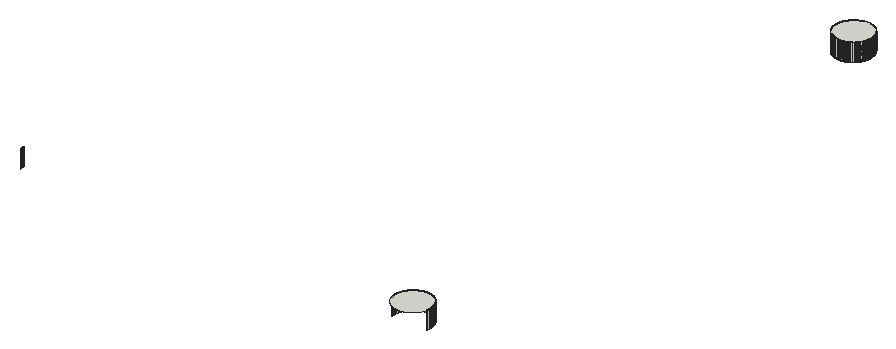
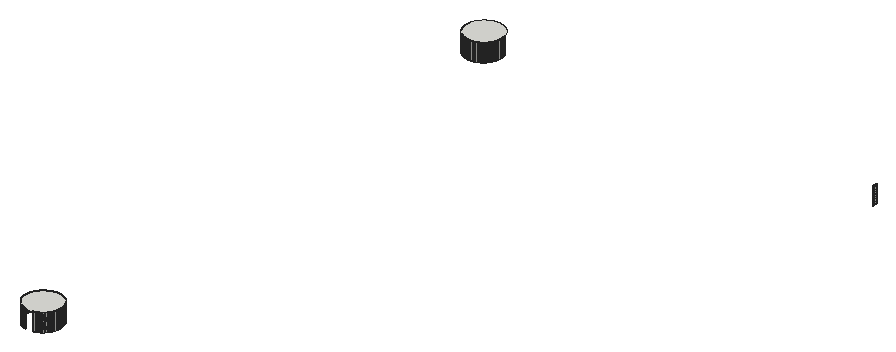
# SketchUp Ruby script. Lengths in inches.
U = 1.inch
M = Sketchup.active_model
def pt(a) = Geom::Point3d.new(a.map { |v| v * U })
def face(e, loops, mat)
  f = e.add_face(loops[0].map { |a| pt(a) })
  loops[1..].each { |l| e.add_face(l.map { |a| pt(a) }).erase! }
  f.material = f.back_material = mat if mat
  f
end
# faces: each face lists its corners as indices into pts; further lists are holes
def faces(e, pts, list, mat = nil) = list.each { |f| face(e, (f[0].is_a?(Array) ? f : [f]).map { |l| l.map { |i| pts[i] } }, mat) }
# xy, xz, yz: faces in a plane at the given z, y or x. An outline is a flat list of corners, or four numbers for a rectangle; further outlines are holes
def ring(l) = l.size == 4 ? [[l[0], l[1]], [l[2], l[1]], [l[2], l[3]], [l[0], l[3]]] : l.each_slice(2).to_a
def flat(e, list, mat, &to3) = list.each { |f| face(e, (f[0].is_a?(Array) ? f : [f]).map { |l| ring(l).map { |u, v| to3.(u, v) } }, mat) }
def xy(e, z, list, mat = nil) = flat(e, list, mat) { |x, y| [x, y, z] }
def xz(e, y, list, mat = nil) = flat(e, list, mat) { |x, z| [x, y, z] }
def yz(e, x, list, mat = nil) = flat(e, list, mat) { |y, z| [x, y, z] }
def lines(e, pts, list) = list.each { |a, b| e.add_line(pt(pts[a]), pt(pts[b])) }
# prism: a flat outline (further loops are holes) pulled along v
def prism(e, loops, v, mat = nil)
  f = face(e, loops, mat); d = Geom::Vector3d.new(v.map { |x| x * U })
  f.pushpull(f.normal.samedirection?(d) ? d.length : -d.length)
end
def box(e, o, s, mat = nil) = prism(e, [[o, [o[0] + s[0], o[1], o[2]], [o[0] + s[0], o[1] + s[1], o[2]], [o[0], o[1] + s[1], o[2]]]], [0, 0, s[2]], mat)
def at(x, y, z, deg = 0) = Geom::Transformation.translation(pt([x, y, z])) * Geom::Transformation.rotation(ORIGIN, Z_AXIS, deg.degrees)
def axes(o, x, y, z) = Geom::Transformation.new([*x, 0, *y, 0, *z, 0, *pt(o).to_a, 1])
def part(name) = M.definitions.add(name)
# library, detail: a bought-in or finely detailed component or shape, given as its bounding box
def library(name, o, s) = part(name).tap { |d| box(d.entities, o, s) }
def detail(e, o, s) = box(e.add_group.entities, o, s)
def put(e, d, t, mat = nil) = e.add_instance(d, t).tap { |i| i.material = mat if mat }
def group(e, t, mat = nil) = e.add_group.tap { |g| g.transformation = t; g.material = mat if mat }.entities
root = M.entities
xy(root,351,[[251.84,249,251.76,249.01,251.6875,249.02,251.61,249.03,251.45,249.05,251.375,249.07,251.3,249.08,251.22,249.1,251.15,249.125,251.07,249.15,251,249.17,250.92,249.2,250.71,249.29,250.64,249.33,250.57,249.36,250.43,249.44,250.37,249.48,250.3,249.53,250.24,249.57,250.17,249.62,249.93,249.82,249.88,249.88,249.77,249.99,249.62,250.17,249.57,250.24,249.53,250.3,249.48,250.37,249.44,250.43,249.36,250.57,249.33,250.64,249.29,250.71,249.23,250.85,249.2,250.93,249.17,251,249.15,251.07,249.125,251.15,249.1,251.22,249.08,251.3,249.07,251.375,249.05,251.45,249.03,251.61,249.02,251.6875,249.01,251.76,249,251.84,249,252.16,249.01,252.24,249.02,252.3125,249.03,252.39,249.05,252.55,249.07,252.625,249.08,252.7,249.1,252.78,249.125,252.85,249.15,252.93,249.17,253,249.2,253.08,249.29,253.29,249.33,253.36,249.36,253.43,249.44,253.57,249.48,253.63,249.53,253.7,249.57,253.76,249.62,253.83,249.82,254.07,249.88,254.12,249.99,254.23,250.17,254.38,250.24,254.43,250.3,254.47,250.37,254.52,250.43,254.56,250.57,254.64,250.64,254.67,250.71,254.71,250.85,254.77,250.93,254.8,251,254.83,251.07,254.85,251.15,254.875,251.22,254.9,251.3,254.92,251.375,254.93,251.45,254.95,251.61,254.97,251.6875,254.98,251.76,254.99,251.84,255,252.16,255,252.24,254.99,252.3125,254.98,252.39,254.97,252.55,254.95,252.625,254.93,252.7,254.92,252.78,254.9,252.85,254.875,252.93,254.85,253,254.83,253.08,254.8,253.29,254.71,253.36,254.67,253.43,254.64,253.57,254.56,253.63,254.52,253.7,254.47,253.76,254.43,253.83,254.38,254.07,254.18,254.12,254.12,254.23,254.01,254.38,253.83,254.43,253.76,254.47,253.7,254.52,253.63,254.56,253.57,254.64,253.43,254.67,253.36,254.71,253.29,254.77,253.15,254.8,253.07,254.83,253,254.85,252.93,254.875,252.85,254.9,252.78,254.92,252.7,254.93,252.625,254.95,252.55,254.97,252.39,254.98,252.3125,254.99,252.24,255,252.16,255,251.84,254.99,251.76,254.98,251.6875,254.97,251.61,254.95,251.45,254.93,251.375,254.92,251.3,254.9,251.22,254.875,251.15,254.85,251.07,254.83,251,254.8,250.92,254.71,250.71,254.67,250.64,254.64,250.57,254.56,250.43,254.52,250.37,254.47,250.3,254.43,250.24,254.38,250.17,254.18,249.93,254.12,249.88,254.01,249.77,253.83,249.62,253.76,249.57,253.7,249.53,253.63,249.48,253.57,249.44,253.43,249.36,253.36,249.33,253.29,249.29,253.15,249.23,253.07,249.2,253,249.17,252.93,249.15,252.85,249.125,252.78,249.1,252.7,249.08,252.625,249.07,252.55,249.05,252.39,249.03,252.3125,249.02,252.24,249.01,252.16,249],[251.84,342,251.76,342.01,251.6875,342.02,251.61,342.03,251.45,342.05,251.375,342.07,251.3,342.08,251.22,342.1,251.15,342.125,251.07,342.15,251,342.17,250.92,342.2,250.71,342.29,250.64,342.33,250.57,342.36,250.43,342.44,250.37,342.48,250.3,342.53,250.24,342.57,250.17,342.62,249.93,342.82,249.88,342.88,249.77,342.99,249.62,343.17,249.57,343.24,249.53,343.3,249.48,343.37,249.44,343.43,249.36,343.57,249.33,343.64,249.29,343.71,249.23,343.85,249.2,343.93,249.17,344,249.15,344.07,249.125,344.15,249.1,344.22,249.08,344.3,249.07,344.375,249.05,344.45,249.03,344.61,249.02,344.6875,249.01,344.76,249,344.84,249,345.16,249.01,345.24,249.02,345.3125,249.03,345.39,249.05,345.55,249.07,345.625,249.08,345.7,249.1,345.78,249.125,345.85,249.15,345.93,249.17,346,249.2,346.08,249.29,346.29,249.33,346.36,249.36,346.43,249.44,346.57,249.48,346.63,249.53,346.7,249.57,346.76,249.62,346.83,249.82,347.07,249.88,347.12,249.99,347.23,250.17,347.38,250.24,347.43,250.3,347.47,250.37,347.52,250.43,347.56,250.57,347.64,250.64,347.67,250.71,347.71,250.85,347.77,250.93,347.8,251,347.83,251.07,347.85,251.15,347.875,251.22,347.9,251.3,347.92,251.375,347.93,251.45,347.95,251.61,347.97,251.6875,347.98,251.76,347.99,251.84,348,252.16,348,252.24,347.99,252.3125,347.98,252.39,347.97,252.55,347.95,252.625,347.93,252.7,347.92,252.78,347.9,252.85,347.875,252.93,347.85,253,347.83,253.08,347.8,253.29,347.71,253.36,347.67,253.43,347.64,253.57,347.56,253.63,347.52,253.7,347.47,253.76,347.43,253.83,347.38,254.07,347.18,254.12,347.12,254.23,347.01,254.38,346.83,254.43,346.76,254.47,346.7,254.52,346.63,254.56,346.57,254.64,346.43,254.67,346.36,254.71,346.29,254.77,346.15,254.8,346.07,254.83,346,254.85,345.93,254.875,345.85,254.9,345.78,254.92,345.7,254.93,345.625,254.95,345.55,254.97,345.39,254.98,345.3125,254.99,345.24,255,345.16,255,344.84,254.99,344.76,254.98,344.6875,254.97,344.61,254.95,344.45,254.93,344.375,254.92,344.3,254.9,344.22,254.875,344.15,254.85,344.07,254.83,344,254.8,343.92,254.71,343.71,254.67,343.64,254.64,343.57,254.56,343.43,254.52,343.37,254.47,343.3,254.43,343.24,254.38,343.17,254.18,342.93,254.12,342.88,254.01,342.77,253.83,342.62,253.76,342.57,253.7,342.53,253.63,342.48,253.57,342.44,253.43,342.36,253.36,342.33,253.29,342.29,253.15,342.23,253.07,342.2,253,342.17,252.93,342.15,252.85,342.125,252.78,342.1,252.7,342.08,252.625,342.07,252.55,342.05,252.39,342.03,252.3125,342.02,252.24,342.01,252.16,342]])
xz(root,255,[[251.84,348,251.92,351],[251.92,348,252,351],[252,348,252.08,351],[252.08,348,252.16,351]])
xz(root,342,[[251.84,348,251.92,351],[251.92,348,252,351],[252,348,252.08,351],[252.08,348,252.16,351]])
yz(root,186,[[251.84,348,251.92,351],[251.92,348,252,351],[252,348,252.08,351],[252.08,348,252.16,351]])
yz(root,249,[[251.84,348,251.92,351],[251.92,348,252,351],[252,348,252.08,351],[252.08,348,252.16,351],[344.84,348,344.92,351],
  [344.92,348,345,351],[345,348,345.08,351],[345.08,348,345.16,351]])
yz(root,255,[[251.84,348,251.92,351],[251.92,348,252,351],[252,348,252.08,351],[252.08,348,252.16,351],[344.84,348,344.92,351],
  [344.92,348,345,351],[345,348,345.08,351],[345.08,348,345.16,351]])
p = [[249.08,251.3,348],[249.07,251.375,348],[249.07,251.375,351],[249.08,251.3,351],[249.05,251.45,348],[249.05,251.45,351],
  [254.95,251.45,348],[254.93,251.375,348],[254.93,251.375,351],[254.95,251.45,351],[249.04,251.53,348],[249.03,251.61,348],
  [249.03,251.61,351],[249.04,251.53,351],[254.96,251.53,348],[254.96,251.53,351],[254.97,251.61,348],[254.97,251.61,351],
  [249.02,251.6875,348],[249.02,251.6875,351],[254.98,251.6875,348],[254.98,251.6875,351],[185.99,251.76,348],[185.98,251.6875,348],
  [185.98,251.6875,351],[185.99,251.76,351],[249.01,251.76,348],[249.01,251.76,351],[254.99,251.76,348],[254.99,251.76,351],
  [186,251.84,348],[186,251.84,351],[249,251.84,348],[249,251.84,351],[255,251.84,348],[255,251.84,351],
  [185.98,252.3125,348],[185.99,252.24,348],[185.99,252.24,351],[185.98,252.3125,351],[186,252.16,348],[186,252.16,351],
  [249,252.16,348],[249.01,252.24,348],[249.01,252.24,351],[249,252.16,351],[249.02,252.3125,348],[249.02,252.3125,351],
  [254.98,252.3125,348],[254.99,252.24,348],[254.99,252.24,351],[254.98,252.3125,351],[255,252.16,348],[255,252.16,351],
  [185.97,252.39,348],[185.97,252.39,351],[249.03,252.39,348],[249.03,252.39,351],[254.97,252.39,348],[254.97,252.39,351],
  [249.04,252.47,348],[249.04,252.47,351],[254.96,252.47,348],[254.96,252.47,351],[249.05,252.55,348],[249.05,252.55,351],
  [249.07,252.625,348],[249.07,252.625,351],[254.93,252.625,348],[254.95,252.55,348],[254.95,252.55,351],[254.93,252.625,351],
  [249.08,252.7,348],[249.08,252.7,351],[254.92,252.7,348],[254.92,252.7,351],[249.1,252.78,348],[249.1,252.78,351],
  [254.9,252.78,348],[254.9,252.78,351],[249.125,252.85,348],[249.125,252.85,351],[254.875,252.85,348],[254.875,252.85,351],
  [249.15,252.93,348],[249.15,252.93,351],[249.17,253,348],[249.17,253,351],[254.83,253,348],[254.85,252.93,348],
  [254.85,252.93,351],[254.83,253,351],[249.2,253.08,348],[249.2,253.08,351],[254.8,253.07,348],[254.8,253.07,351],
  [249.23,253.15,348],[249.23,253.15,351],[249.26,253.22,348],[249.26,253.22,351],[254.74,253.22,348],[254.77,253.15,348],
  [254.77,253.15,351],[254.74,253.22,351],[249.29,253.29,348],[249.29,253.29,351],[254.71,253.29,348],[254.71,253.29,351],
  [249.33,253.36,348],[249.33,253.36,351],[254.67,253.36,348],[254.67,253.36,351],[249.36,253.43,348],[249.36,253.43,351],
  [249.4,253.5,348],[249.4,253.5,351],[254.6,253.5,348],[254.64,253.43,348],[254.64,253.43,351],[254.6,253.5,351],
  [249.44,253.57,348],[249.44,253.57,351],[254.56,253.57,348],[254.56,253.57,351],[249.48,253.63,348],[249.48,253.63,351],
  [249.53,253.7,348],[249.53,253.7,351],[254.47,253.7,348],[254.52,253.63,348],[254.52,253.63,351],[254.47,253.7,351],
  [249.57,253.76,348],[249.57,253.76,351],[254.43,253.76,348],[254.43,253.76,351],[249.62,253.83,348],[249.62,253.83,351],
  [249.67,253.89,348],[249.67,253.89,351],[254.33,253.89,348],[254.38,253.83,348],[254.38,253.83,351],[254.33,253.89,351],
  [249.72,253.95,348],[249.72,253.95,351],[249.77,254.01,348],[249.77,254.01,351],[254.23,254.01,348],[254.28,253.95,348],
  [254.28,253.95,351],[254.23,254.01,351],[249.82,254.07,348],[249.82,254.07,351],[254.18,254.06,348],[254.18,254.06,351],
  [249.88,254.12,348],[249.88,254.12,351],[249.94,254.18,348],[249.94,254.18,351],[254.07,254.18,348],[254.12,254.12,348],
  [254.12,254.12,351],[254.07,254.18,351],[249.99,254.23,348],[249.99,254.23,351],[250.05,254.28,348],[250.05,254.28,351],
  [253.95,254.28,348],[254.01,254.23,348],[254.01,254.23,351],[253.95,254.28,351],[250.11,254.33,348],[250.11,254.33,351],
  [250.17,254.38,348],[250.17,254.38,351],[253.83,254.38,348],[253.89,254.33,348],[253.89,254.33,351],[253.83,254.38,351],
  [250.24,254.43,348],[250.24,254.43,351],[250.3,254.47,348],[250.3,254.47,351],[253.7,254.47,348],[253.76,254.43,348],
  [253.76,254.43,351],[253.7,254.47,351],[250.37,254.52,348],[250.37,254.52,351],[250.43,254.56,348],[250.43,254.56,351],
  [253.57,254.56,348],[253.63,254.52,348],[253.63,254.52,351],[253.57,254.56,351],[250.5,254.6,348],[250.5,254.6,351],
  [250.57,254.64,348],[250.57,254.64,351],[250.64,254.67,348],[250.64,254.67,351],[253.36,254.67,348],[253.43,254.64,348],
  [253.43,254.64,351],[253.36,254.67,351],[253.5,254.6,348],[253.5,254.6,351],[250.71,254.71,348],[250.71,254.71,351],
  [250.78,254.74,348],[250.78,254.74,351],[250.85,254.77,348],[250.85,254.77,351],[253.15,254.77,348],[253.22,254.74,348],
  [253.22,254.74,351],[253.15,254.77,351],[253.29,254.71,348],[253.29,254.71,351],[250.93,254.8,348],[250.93,254.8,351],
  [251,254.83,348],[251,254.83,351],[251.07,254.85,348],[251.07,254.85,351],[252.93,254.85,348],[253,254.83,348],
  [253,254.83,351],[252.93,254.85,351],[253.08,254.8,348],[253.08,254.8,351],[251.15,254.875,348],[251.15,254.875,351],
  [251.22,254.9,348],[251.22,254.9,351],[251.3,254.92,348],[251.3,254.92,351],[251.375,254.93,348],[251.375,254.93,351],
  [251.45,254.95,348],[251.45,254.95,351],[251.53,254.96,348],[251.53,254.96,351],[252.47,254.96,348],[252.55,254.95,348],
  [252.55,254.95,351],[252.47,254.96,351],[252.625,254.93,348],[252.625,254.93,351],[252.7,254.92,348],[252.7,254.92,351],
  [252.78,254.9,348],[252.78,254.9,351],[252.85,254.875,348],[252.85,254.875,351],[251.61,254.97,348],[251.61,254.97,351],
  [251.6875,254.98,348],[251.6875,254.98,351],[251.76,254.99,348],[251.76,254.99,351],[251.84,255,348],[251.84,255,351],
  [252.16,255,348],[252.24,254.99,348],[252.24,254.99,351],[252.16,255,351],[252.3125,254.98,348],[252.3125,254.98,351],
  [252.39,254.97,348],[252.39,254.97,351],[251.53,342.04,348],[251.45,342.05,348],[251.45,342.05,351],[251.53,342.04,351],
  [251.61,342.03,348],[251.61,342.03,351],[251.6875,342.02,348],[251.6875,342.02,351],[251.76,342.01,348],[251.76,342.01,351],
  [251.84,342,348],[251.84,342,351],[252.24,342.01,348],[252.16,342,348],[252.16,342,351],[252.24,342.01,351],
  [252.3125,342.02,348],[252.3125,342.02,351],[252.39,342.03,348],[252.39,342.03,351],[252.47,342.04,348],[252.47,342.04,351],
  [252.55,342.05,348],[252.55,342.05,351],[251.07,342.15,348],[251,342.17,348],[251,342.17,351],[251.07,342.15,351],
  [251.15,342.125,348],[251.15,342.125,351],[251.22,342.1,348],[251.22,342.1,351],[251.3,342.08,348],[251.3,342.08,351],
  [251.375,342.07,348],[251.375,342.07,351],[252.625,342.07,348],[252.625,342.07,351],[252.7,342.08,348],[252.7,342.08,351],
  [252.78,342.1,348],[252.78,342.1,351],[252.85,342.125,348],[252.85,342.125,351],[252.93,342.15,348],[252.93,342.15,351],
  [253,342.17,348],[253,342.17,351],[250.85,342.23,348],[250.78,342.26,348],[250.78,342.26,351],[250.85,342.23,351],
  [250.92,342.2,348],[250.92,342.2,351],[253.07,342.2,348],[253.07,342.2,351],[253.15,342.23,348],[253.15,342.23,351],
  [253.22,342.26,348],[253.22,342.26,351],[250.64,342.33,348],[250.57,342.36,348],[250.57,342.36,351],[250.64,342.33,351],
  [250.71,342.29,348],[250.71,342.29,351],[253.29,342.29,348],[253.29,342.29,351],[253.36,342.33,348],[253.36,342.33,351],
  [253.43,342.36,348],[253.43,342.36,351],[250.43,342.44,348],[250.37,342.48,348],[250.37,342.48,351],[250.43,342.44,351],
  [250.5,342.4,348],[250.5,342.4,351],[253.5,342.4,348],[253.5,342.4,351],[253.57,342.44,348],[253.57,342.44,351],
  [253.63,342.48,348],[253.63,342.48,351],[250.3,342.53,348],[250.24,342.57,348],[250.24,342.57,351],[250.3,342.53,351],
  [253.7,342.53,348],[253.7,342.53,351],[253.76,342.57,348],[253.76,342.57,351],[250.17,342.62,348],[250.11,342.67,348],
  [250.11,342.67,351],[250.17,342.62,351],[253.83,342.62,348],[253.83,342.62,351],[253.89,342.67,348],[253.89,342.67,351],
  [250.05,342.72,348],[249.99,342.77,348],[249.99,342.77,351],[250.05,342.72,351],[253.95,342.72,348],[253.95,342.72,351],
  [254.01,342.77,348],[254.01,342.77,351],[249.93,342.82,348],[249.88,342.88,348],[249.88,342.88,351],[249.93,342.82,351],
  [254.06,342.82,348],[254.06,342.82,351],[254.12,342.88,348],[254.12,342.88,351],[249.82,342.94,348],[249.77,342.99,348],
  [249.77,342.99,351],[249.82,342.94,351],[254.18,342.93,348],[254.18,342.93,351],[254.23,342.99,348],[254.23,342.99,351],
  [249.72,343.05,348],[249.72,343.05,351],[254.28,343.05,348],[254.28,343.05,351],[249.67,343.11,348],[249.62,343.17,348],
  [249.62,343.17,351],[249.67,343.11,351],[254.33,343.11,348],[254.33,343.11,351],[254.38,343.17,348],[254.38,343.17,351],
  [249.57,343.24,348],[249.53,343.3,348],[249.53,343.3,351],[249.57,343.24,351],[254.43,343.24,348],[254.43,343.24,351],
  [254.47,343.3,348],[254.47,343.3,351],[249.48,343.37,348],[249.48,343.37,351],[254.52,343.37,348],[254.52,343.37,351],
  [249.44,343.43,348],[249.4,343.5,348],[249.4,343.5,351],[249.44,343.43,351],[254.56,343.43,348],[254.56,343.43,351],
  [254.6,343.5,348],[254.6,343.5,351],[249.36,343.57,348],[249.36,343.57,351],[254.64,343.57,348],[254.64,343.57,351],
  [249.33,343.64,348],[249.29,343.71,348],[249.29,343.71,351],[249.33,343.64,351],[254.67,343.64,348],[254.67,343.64,351],
  [254.71,343.71,348],[254.71,343.71,351],[249.26,343.78,348],[249.26,343.78,351],[254.74,343.78,348],[254.74,343.78,351],
  [249.23,343.85,348],[249.23,343.85,351],[254.77,343.85,348],[254.77,343.85,351],[249.2,343.93,348],[249.17,344,348],
  [249.17,344,351],[249.2,343.93,351],[254.8,343.92,348],[254.8,343.92,351],[254.83,344,348],[254.83,344,351],
  [249.15,344.07,348],[249.15,344.07,351],[254.85,344.07,348],[254.85,344.07,351],[249.125,344.15,348],[249.1,344.22,348],
  [249.1,344.22,351],[249.125,344.15,351],[254.875,344.15,348],[254.875,344.15,351],[254.9,344.22,348],[254.9,344.22,351],
  [249.08,344.3,348],[249.08,344.3,351],[254.92,344.3,348],[254.92,344.3,351],[249.07,344.375,348],[249.07,344.375,351],
  [254.93,344.375,348],[254.93,344.375,351],[249.05,344.45,348],[249.05,344.45,351],[254.95,344.45,348],[254.95,344.45,351],
  [249.04,344.53,348],[249.03,344.61,348],[249.03,344.61,351],[249.04,344.53,351],[254.96,344.53,348],[254.96,344.53,351],
  [254.97,344.61,348],[254.97,344.61,351],[249.02,344.6875,348],[249.02,344.6875,351],[254.98,344.6875,348],[254.98,344.6875,351],
  [249.01,344.76,348],[249.01,344.76,351],[254.99,344.76,348],[254.99,344.76,351],[249,344.84,348],[249,344.84,351],
  [255,344.84,348],[255,344.84,351],[249,345.16,348],[249.01,345.24,348],[249.01,345.24,351],[249,345.16,351],
  [249.02,345.3125,348],[249.02,345.3125,351],[254.98,345.3125,348],[254.99,345.24,348],[254.99,345.24,351],[254.98,345.3125,351],
  [255,345.16,348],[255,345.16,351],[249.03,345.39,348],[249.03,345.39,351],[254.97,345.39,348],[254.97,345.39,351],
  [249.04,345.47,348],[249.04,345.47,351],[254.96,345.47,348],[254.96,345.47,351],[249.05,345.55,348],[249.05,345.55,351],
  [249.07,345.625,348],[249.07,345.625,351],[254.93,345.625,348],[254.95,345.55,348],[254.95,345.55,351],[254.93,345.625,351],
  [249.08,345.7,348],[249.08,345.7,351],[254.92,345.7,348],[254.92,345.7,351],[249.1,345.78,348],[249.1,345.78,351],
  [254.9,345.78,348],[254.9,345.78,351],[249.125,345.85,348],[249.125,345.85,351],[254.875,345.85,348],[254.875,345.85,351],
  [249.15,345.93,348],[249.15,345.93,351],[249.17,346,348],[249.17,346,351],[254.83,346,348],[254.85,345.93,348],
  [254.85,345.93,351],[254.83,346,351],[249.2,346.08,348],[249.2,346.08,351],[254.8,346.07,348],[254.8,346.07,351],
  [249.23,346.15,348],[249.23,346.15,351],[249.26,346.22,348],[249.26,346.22,351],[254.74,346.22,348],[254.77,346.15,348],
  [254.77,346.15,351],[254.74,346.22,351],[249.29,346.29,348],[249.29,346.29,351],[254.71,346.29,348],[254.71,346.29,351],
  [249.33,346.36,348],[249.33,346.36,351],[254.67,346.36,348],[254.67,346.36,351],[249.36,346.43,348],[249.36,346.43,351],
  [249.4,346.5,348],[249.4,346.5,351],[254.6,346.5,348],[254.64,346.43,348],[254.64,346.43,351],[254.6,346.5,351],
  [249.44,346.57,348],[249.44,346.57,351],[254.56,346.57,348],[254.56,346.57,351],[249.48,346.63,348],[249.48,346.63,351],
  [249.53,346.7,348],[249.53,346.7,351],[254.47,346.7,348],[254.52,346.63,348],[254.52,346.63,351],[254.47,346.7,351],
  [249.57,346.76,348],[249.57,346.76,351],[254.43,346.76,348],[254.43,346.76,351],[249.62,346.83,348],[249.62,346.83,351],
  [249.67,346.89,348],[249.67,346.89,351],[254.33,346.89,348],[254.38,346.83,348],[254.38,346.83,351],[254.33,346.89,351],
  [249.72,346.95,348],[249.72,346.95,351],[249.77,347.01,348],[249.77,347.01,351],[254.23,347.01,348],[254.28,346.95,348],
  [254.28,346.95,351],[254.23,347.01,351],[249.82,347.07,348],[249.82,347.07,351],[254.18,347.06,348],[254.18,347.06,351],
  [249.88,347.12,348],[249.88,347.12,351],[249.94,347.18,348],[249.94,347.18,351],[254.07,347.18,348],[254.12,347.12,348],
  [254.12,347.12,351],[254.07,347.18,351],[249.99,347.23,348],[249.99,347.23,351],[250.05,347.28,348],[250.05,347.28,351],
  [253.95,347.28,348],[254.01,347.23,348],[254.01,347.23,351],[253.95,347.28,351],[250.11,347.33,348],[250.11,347.33,351],
  [250.17,347.38,348],[250.17,347.38,351],[253.83,347.38,348],[253.89,347.33,348],[253.89,347.33,351],[253.83,347.38,351],
  [250.24,347.43,348],[250.24,347.43,351],[250.3,347.47,348],[250.3,347.47,351],[253.7,347.47,348],[253.76,347.43,348],
  [253.76,347.43,351],[253.7,347.47,351],[250.37,347.52,348],[250.37,347.52,351],[250.43,347.56,348],[250.43,347.56,351],
  [253.57,347.56,348],[253.63,347.52,348],[253.63,347.52,351],[253.57,347.56,351],[250.5,347.6,348],[250.5,347.6,351],
  [250.57,347.64,348],[250.57,347.64,351],[250.64,347.67,348],[250.64,347.67,351],[253.36,347.67,348],[253.43,347.64,348],
  [253.43,347.64,351],[253.36,347.67,351],[253.5,347.6,348],[253.5,347.6,351],[250.71,347.71,348],[250.71,347.71,351],
  [250.78,347.74,348],[250.78,347.74,351],[250.85,347.77,348],[250.85,347.77,351],[253.15,347.77,348],[253.22,347.74,348],
  [253.22,347.74,351],[253.15,347.77,351],[253.29,347.71,348],[253.29,347.71,351],[250.93,347.8,348],[250.93,347.8,351],
  [251,347.83,348],[251,347.83,351],[251.07,347.85,348],[251.07,347.85,351],[252.93,347.85,348],[253,347.83,348],
  [253,347.83,351],[252.93,347.85,351],[253.08,347.8,348],[253.08,347.8,351],[251.15,347.875,348],[251.15,347.875,351],
  [251.22,347.9,348],[251.22,347.9,351],[251.3,347.92,348],[251.3,347.92,351],[251.375,347.93,348],[251.375,347.93,351],
  [251.45,347.95,348],[251.45,347.95,351],[252.47,347.96,348],[252.55,347.95,348],[252.55,347.95,351],[252.47,347.96,351],
  [252.625,347.93,348],[252.625,347.93,351],[252.7,347.92,348],[252.7,347.92,351],[252.78,347.9,348],[252.78,347.9,351],
  [252.85,347.875,348],[252.85,347.875,351]]
faces(root,p,[[0,1,2,3],[1,4,5,2],[6,7,8,9],[10,11,12,13],[4,10,13,5],[14,6,9,15],[16,14,15,17],[11,18,19,12],
  [20,16,17,21],[22,23,24,25],[18,26,27,19],[28,20,21,29],[30,22,25,31],[26,32,33,27],[34,28,29,35],[36,37,38,39],
  [37,40,41,38],[42,43,44,45],[43,46,47,44],[48,49,50,51],[49,52,53,50],[54,36,39,55],[46,56,57,47],[58,48,51,59],
  [56,60,61,57],[62,58,59,63],[60,64,65,61],[64,66,67,65],[68,69,70,71],[69,62,63,70],[66,72,73,67],[74,68,71,75],
  [72,76,77,73],[78,74,75,79],[76,80,81,77],[82,78,79,83],[80,84,85,81],[84,86,87,85],[88,89,90,91],[89,82,83,90],
  [86,92,93,87],[94,88,91,95],[92,96,97,93],[96,98,99,97],[100,101,102,103],[101,94,95,102],[98,104,105,99],[106,100,103,107],
  [104,108,109,105],[110,106,107,111],[108,112,113,109],[112,114,115,113],[116,117,118,119],[117,110,111,118],[114,120,121,115],[122,116,119,123],
  [120,124,125,121],[124,126,127,125],[128,129,130,131],[129,122,123,130],[126,132,133,127],[134,128,131,135],[132,136,137,133],[136,138,139,137],
  [140,141,142,143],[141,134,135,142],[138,144,145,139],[144,146,147,145],[148,149,150,151],[149,140,143,150],[146,152,153,147],[154,148,151,155],
  [152,156,157,153],[156,158,159,157],[160,161,162,163],[161,154,155,162],[158,164,165,159],[164,166,167,165],[168,169,170,171],[169,160,163,170],
  [166,172,173,167],[172,174,175,173],[176,177,178,179],[177,168,171,178],[174,180,181,175],[180,182,183,181],[184,185,186,187],[185,176,179,186],
  [182,188,189,183],[188,190,191,189],[192,193,194,195],[193,184,187,194],[190,196,197,191],[196,198,199,197],[198,200,201,199],[202,203,204,205],
  [203,206,207,204],[206,192,195,207],[200,208,209,201],[208,210,211,209],[210,212,213,211],[214,215,216,217],[215,218,219,216],[218,202,205,219],
  [212,220,221,213],[220,222,223,221],[222,224,225,223],[226,227,228,229],[227,230,231,228],[230,214,217,231],[224,232,233,225],[232,234,235,233],
  [234,236,237,235],[236,238,239,237],[238,240,241,239],[240,242,243,241],[244,245,246,247],[245,248,249,246],[248,250,251,249],[250,252,253,251],
  [252,254,255,253],[254,226,229,255],[242,256,257,243],[256,258,259,257],[258,260,261,259],[260,262,263,261],[264,265,266,267],[265,268,269,266],
  [268,270,271,269],[270,244,247,271],[272,273,274,275],[276,272,275,277],[278,276,277,279],[280,278,279,281],[282,280,281,283],[284,285,286,287],
  [288,284,287,289],[290,288,289,291],[292,290,291,293],[294,292,293,295],[296,297,298,299],[300,296,299,301],[302,300,301,303],[304,302,303,305],
  [306,304,305,307],[273,306,307,274],[308,294,295,309],[310,308,309,311],[312,310,311,313],[314,312,313,315],[316,314,315,317],[318,316,317,319],
  [320,321,322,323],[324,320,323,325],[297,324,325,298],[326,318,319,327],[328,326,327,329],[330,328,329,331],[332,333,334,335],[336,332,335,337],
  [321,336,337,322],[338,330,331,339],[340,338,339,341],[342,340,341,343],[344,345,346,347],[348,344,347,349],[333,348,349,334],[350,342,343,351],
  [352,350,351,353],[354,352,353,355],[356,357,358,359],[345,356,359,346],[360,354,355,361],[362,360,361,363],[364,365,366,367],[357,364,367,358],
  [368,362,363,369],[370,368,369,371],[372,373,374,375],[365,372,375,366],[376,370,371,377],[378,376,377,379],[380,381,382,383],[373,380,383,374],
  [384,378,379,385],[386,384,385,387],[388,389,390,391],[381,388,391,382],[392,386,387,393],[394,392,393,395],[389,396,397,390],[398,394,395,399],
  [400,401,402,403],[396,400,403,397],[404,398,399,405],[406,404,405,407],[408,409,410,411],[401,408,411,402],[412,406,407,413],[414,412,413,415],
  [409,416,417,410],[418,414,415,419],[420,421,422,423],[416,420,423,417],[424,418,419,425],[426,424,425,427],[421,428,429,422],[430,426,427,431],
  [432,433,434,435],[428,432,435,429],[436,430,431,437],[438,436,437,439],[433,440,441,434],[442,438,439,443],[440,444,445,441],[446,442,443,447],
  [448,449,450,451],[444,448,451,445],[452,446,447,453],[454,452,453,455],[449,456,457,450],[458,454,455,459],[460,461,462,463],[456,460,463,457],
  [464,458,459,465],[466,464,465,467],[461,468,469,462],[470,466,467,471],[468,472,473,469],[474,470,471,475],[472,476,477,473],[478,474,475,479],
  [480,481,482,483],[476,480,483,477],[484,478,479,485],[486,484,485,487],[481,488,489,482],[490,486,487,491],[488,492,493,489],[494,490,491,495],
  [492,496,497,493],[498,494,495,499],[500,501,502,503],[501,504,505,502],[506,507,508,509],[507,510,511,508],[504,512,513,505],[514,506,509,515],
  [512,516,517,513],[518,514,515,519],[516,520,521,517],[520,522,523,521],[524,525,526,527],[525,518,519,526],[522,528,529,523],[530,524,527,531],
  [528,532,533,529],[534,530,531,535],[532,536,537,533],[538,534,535,539],[536,540,541,537],[540,542,543,541],[544,545,546,547],[545,538,539,546],
  [542,548,549,543],[550,544,547,551],[548,552,553,549],[552,554,555,553],[556,557,558,559],[557,550,551,558],[554,560,561,555],[562,556,559,563],
  [560,564,565,561],[566,562,563,567],[564,568,569,565],[568,570,571,569],[572,573,574,575],[573,566,567,574],[570,576,577,571],[578,572,575,579],
  [576,580,581,577],[580,582,583,581],[584,585,586,587],[585,578,579,586],[582,588,589,583],[590,584,587,591],[588,592,593,589],[592,594,595,593],
  [596,597,598,599],[597,590,591,598],[594,600,601,595],[600,602,603,601],[604,605,606,607],[605,596,599,606],[602,608,609,603],[610,604,607,611],
  [608,612,613,609],[612,614,615,613],[616,617,618,619],[617,610,611,618],[614,620,621,615],[620,622,623,621],[624,625,626,627],[625,616,619,626],
  [622,628,629,623],[628,630,631,629],[632,633,634,635],[633,624,627,634],[630,636,637,631],[636,638,639,637],[640,641,642,643],[641,632,635,642],
  [638,644,645,639],[644,646,647,645],[648,649,650,651],[649,640,643,650],[646,652,653,647],[652,654,655,653],[654,656,657,655],[658,659,660,661],
  [659,662,663,660],[662,648,651,663],[656,664,665,657],[664,666,667,665],[666,668,669,667],[670,671,672,673],[671,674,675,672],[674,658,661,675],
  [668,676,677,669],[676,678,679,677],[678,680,681,679],[682,683,684,685],[683,686,687,684],[686,670,673,687],[680,688,689,681],[688,690,691,689],
  [690,692,693,691],[692,694,695,693],[694,696,697,695],[698,699,700,701],[699,702,703,700],[702,704,705,703],[704,706,707,705],[706,708,709,707],
  [708,682,685,709]])
